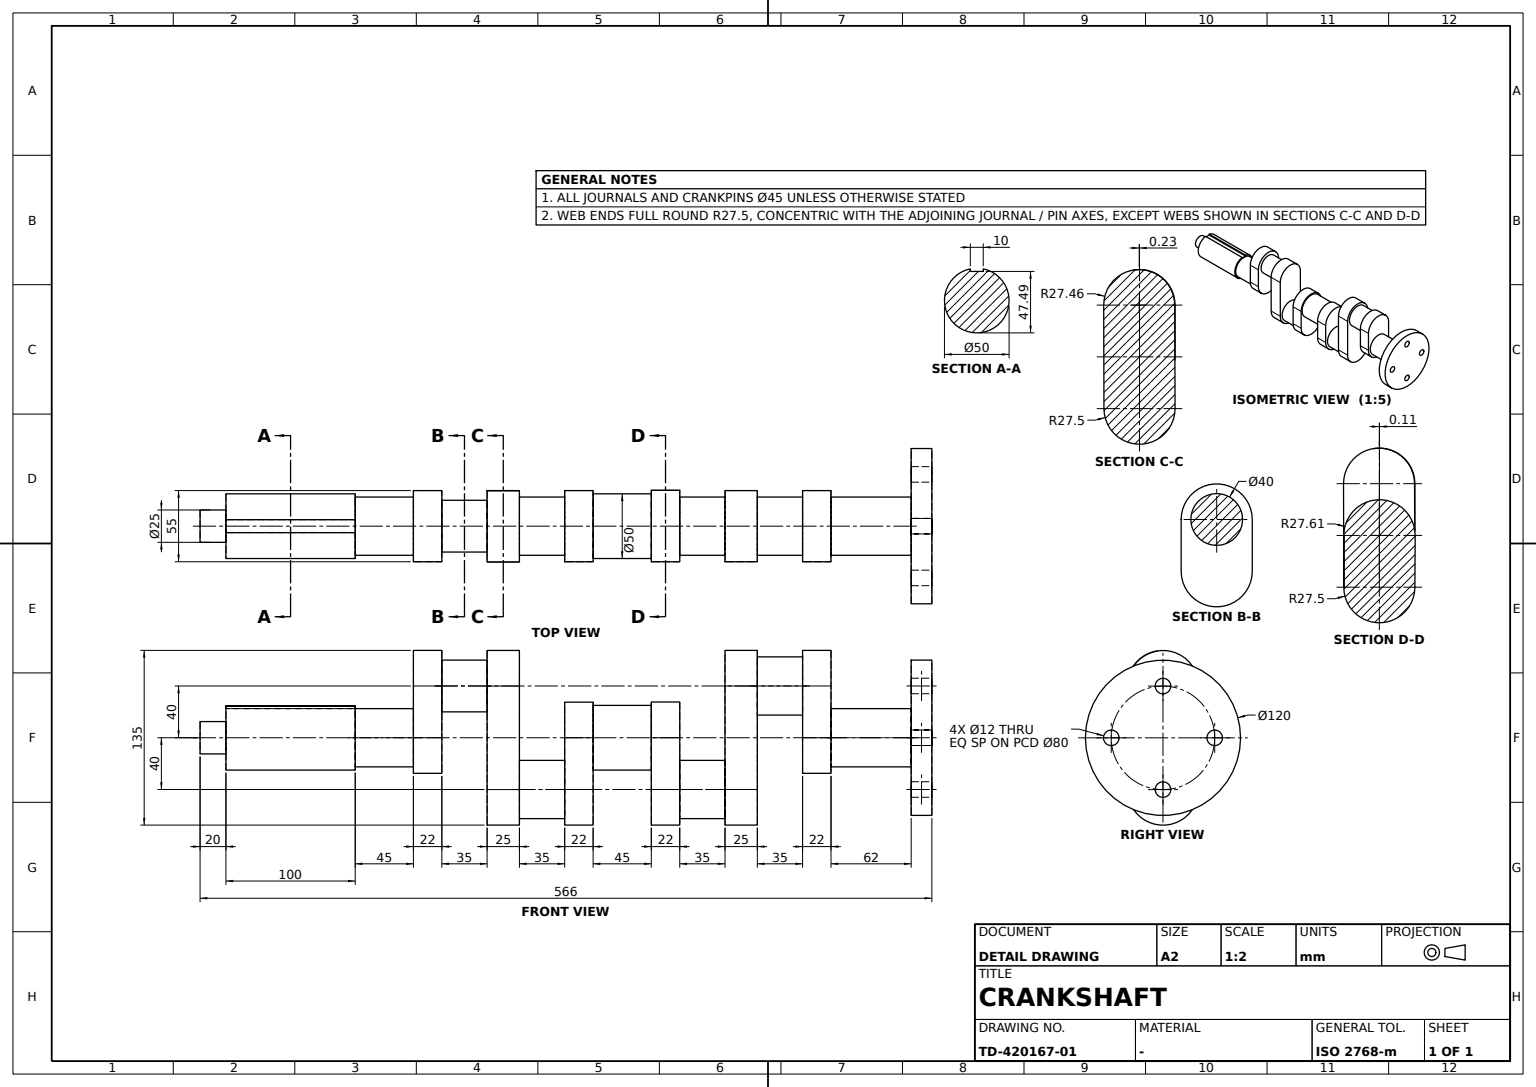
ISO-10303-21;
HEADER;
FILE_DESCRIPTION((''),'2;1');
FILE_NAME('','',(''),(''),'','','');
FILE_SCHEMA(('AUTOMOTIVE_DESIGN'));
ENDSEC;
DATA;
#1=APPLICATION_CONTEXT('');
#2=PRODUCT_CONTEXT('',#1,'mechanical');
#3=PRODUCT('','','',(#2));
#4=PRODUCT_DEFINITION_FORMATION('','',#3);
#5=PRODUCT_DEFINITION_CONTEXT('',#1,'design');
#6=PRODUCT_DEFINITION('','',#4,#5);
#7=PRODUCT_DEFINITION_SHAPE('','',#6);
#8=(LENGTH_UNIT()NAMED_UNIT(*)SI_UNIT(.MILLI.,.METRE.));
#9=(NAMED_UNIT(*)PLANE_ANGLE_UNIT()SI_UNIT($,.RADIAN.));
#10=(NAMED_UNIT(*)SI_UNIT($,.STERADIAN.)SOLID_ANGLE_UNIT());
#11=UNCERTAINTY_MEASURE_WITH_UNIT(LENGTH_MEASURE(0.005),#8,'distance_accuracy_value','');
#12=(GEOMETRIC_REPRESENTATION_CONTEXT(3)GLOBAL_UNCERTAINTY_ASSIGNED_CONTEXT((#11))GLOBAL_UNIT_ASSIGNED_CONTEXT((#8,#9,#10))REPRESENTATION_CONTEXT('',''));
#13=CARTESIAN_POINT('',(-438.,24.494897,-5.));
#14=VERTEX_POINT('',#13);
#15=CARTESIAN_POINT('',(-438.,24.494897,5.));
#16=VERTEX_POINT('',#15);
#17=CARTESIAN_POINT('',(-438.,0.,0.));
#18=DIRECTION('',(-1.,0.,0.));
#19=DIRECTION('',(0.,0.,1.));
#20=AXIS2_PLACEMENT_3D('',#17,#18,#19);
#21=CIRCLE('',#20,25.);
#22=EDGE_CURVE('',#14,#16,#21,.T.);
#23=ORIENTED_EDGE('',*,*,#22,.T.);
#24=CARTESIAN_POINT('',(-538.,24.494897,5.));
#25=VERTEX_POINT('',#24);
#26=VECTOR('',#18,1000.);
#27=LINE('',#24,#26);
#28=EDGE_CURVE('',#25,#16,#27,.F.);
#29=ORIENTED_EDGE('',*,*,#28,.F.);
#30=CARTESIAN_POINT('',(-538.,24.494897,-5.));
#31=VERTEX_POINT('',#30);
#32=CARTESIAN_POINT('',(-538.,0.,0.));
#33=AXIS2_PLACEMENT_3D('',#32,#18,#19);
#34=CIRCLE('',#33,25.);
#35=EDGE_CURVE('',#31,#25,#34,.T.);
#36=ORIENTED_EDGE('',*,*,#35,.F.);
#37=LINE('',#30,#26);
#38=EDGE_CURVE('',#31,#14,#37,.F.);
#39=ORIENTED_EDGE('',*,*,#38,.T.);
#40=EDGE_LOOP('',(#23,#29,#36,#39));
#41=FACE_BOUND('',#40,.T.);
#42=CARTESIAN_POINT('',(-231.5,0.,0.));
#43=DIRECTION('',(0.,-1.,0.));
#44=AXIS2_PLACEMENT_3D('',#42,#18,#43);
#45=CYLINDRICAL_SURFACE('',#44,25.);
#46=ADVANCED_FACE('',(#41),#45,.T.);
#47=CARTESIAN_POINT('',(-254.,0.,27.5));
#48=VERTEX_POINT('',#47);
#49=CARTESIAN_POINT('',(-276.,0.,27.5));
#50=VERTEX_POINT('',#49);
#51=CARTESIAN_POINT('',(-81.,0.,27.5));
#52=LINE('',#51,#26);
#53=EDGE_CURVE('',#48,#50,#52,.T.);
#54=ORIENTED_EDGE('',*,*,#53,.T.);
#55=CARTESIAN_POINT('',(-276.,-40.,27.5));
#56=VERTEX_POINT('',#55);
#57=VECTOR('',#43,1000.);
#58=LINE('',#49,#57);
#59=EDGE_CURVE('',#50,#56,#58,.T.);
#60=ORIENTED_EDGE('',*,*,#59,.T.);
#61=CARTESIAN_POINT('',(-254.,-40.,27.5));
#62=VERTEX_POINT('',#61);
#63=CARTESIAN_POINT('',(-139.5,-40.,27.5));
#64=LINE('',#63,#26);
#65=EDGE_CURVE('',#62,#56,#64,.T.);
#66=ORIENTED_EDGE('',*,*,#65,.F.);
#67=LINE('',#47,#57);
#68=EDGE_CURVE('',#48,#62,#67,.T.);
#69=ORIENTED_EDGE('',*,*,#68,.F.);
#70=EDGE_LOOP('',(#54,#60,#66,#69));
#71=FACE_BOUND('',#70,.T.);
#72=CARTESIAN_POINT('',(-70.,0.,27.5));
#73=DIRECTION('',(0.,1.,0.));
#74=AXIS2_PLACEMENT_3D('',#72,#19,#73);
#75=PLANE('',#74);
#76=ADVANCED_FACE('',(#71),#75,.T.);
#77=CARTESIAN_POINT('',(-311.,39.93292,27.694372));
#78=VERTEX_POINT('',#77);
#79=CARTESIAN_POINT('',(-311.,40.09153,-27.232277));
#80=VERTEX_POINT('',#79);
#81=CARTESIAN_POINT('',(-311.,39.999675,0.231011));
#82=AXIS2_PLACEMENT_3D('',#81,#18,#19);
#83=CIRCLE('',#82,27.463442);
#84=EDGE_CURVE('',#78,#80,#83,.T.);
#85=ORIENTED_EDGE('',*,*,#84,.F.);
#86=CARTESIAN_POINT('',(-311.,-40.066843,27.499919));
#87=VERTEX_POINT('',#86);
#88=CARTESIAN_POINT('',(-311.,-0.06708,27.597145));
#89=DIRECTION('',(0.,0.999997046,0.002430665));
#90=VECTOR('',#89,1000.);
#91=LINE('',#88,#90);
#92=EDGE_CURVE('',#87,#78,#91,.T.);
#93=ORIENTED_EDGE('',*,*,#92,.F.);
#94=CARTESIAN_POINT('',(-311.,-39.908023,-27.499846));
#95=VERTEX_POINT('',#94);
#96=CARTESIAN_POINT('',(-311.,-40.,0.));
#97=AXIS2_PLACEMENT_3D('',#96,#18,#19);
#98=CIRCLE('',#97,27.5);
#99=EDGE_CURVE('',#95,#87,#98,.T.);
#100=ORIENTED_EDGE('',*,*,#99,.F.);
#101=CARTESIAN_POINT('',(-311.,0.09153,-27.366062));
#102=DIRECTION('',(0.,0.999994407,0.003344618));
#103=VECTOR('',#102,1000.);
#104=LINE('',#101,#103);
#105=EDGE_CURVE('',#95,#80,#104,.T.);
#106=ORIENTED_EDGE('',*,*,#105,.T.);
#107=EDGE_LOOP('',(#85,#93,#100,#106));
#108=FACE_BOUND('',#107,.T.);
#109=CARTESIAN_POINT('',(-311.,-40.,22.5));
#110=VERTEX_POINT('',#109);
#111=CIRCLE('',#97,22.5);
#112=EDGE_CURVE('',#110,#110,#111,.T.);
#113=ORIENTED_EDGE('',*,*,#112,.T.);
#114=EDGE_LOOP('',(#113));
#115=FACE_BOUND('',#114,.T.);
#116=CARTESIAN_POINT('',(-311.,0.,0.));
#117=AXIS2_PLACEMENT_3D('',#116,#18,#43);
#118=PLANE('',#117);
#119=ADVANCED_FACE('',(#108,#115),#118,.F.);
#120=CARTESIAN_POINT('',(-70.,-0.005103,22.5));
#121=VERTEX_POINT('',#120);
#122=CARTESIAN_POINT('',(-70.,-0.005103,0.));
#123=AXIS2_PLACEMENT_3D('',#122,#18,#19);
#124=CIRCLE('',#123,22.5);
#125=EDGE_CURVE('',#121,#121,#124,.T.);
#126=ORIENTED_EDGE('',*,*,#125,.T.);
#127=EDGE_LOOP('',(#126));
#128=FACE_BOUND('',#127,.T.);
#129=CARTESIAN_POINT('',(-70.,0.,-27.5));
#130=VERTEX_POINT('',#129);
#131=VERTEX_POINT('',#72);
#132=CARTESIAN_POINT('',(-70.,0.,0.));
#133=AXIS2_PLACEMENT_3D('',#132,#18,#19);
#134=CIRCLE('',#133,27.5);
#135=EDGE_CURVE('',#130,#131,#134,.T.);
#136=ORIENTED_EDGE('',*,*,#135,.F.);
#137=CARTESIAN_POINT('',(-70.,40.,-27.5));
#138=VERTEX_POINT('',#137);
#139=VECTOR('',#73,1000.);
#140=LINE('',#129,#139);
#141=EDGE_CURVE('',#130,#138,#140,.T.);
#142=ORIENTED_EDGE('',*,*,#141,.T.);
#143=CARTESIAN_POINT('',(-70.,40.,27.5));
#144=VERTEX_POINT('',#143);
#145=CARTESIAN_POINT('',(-70.,40.,0.));
#146=AXIS2_PLACEMENT_3D('',#145,#18,#19);
#147=CIRCLE('',#146,27.5);
#148=EDGE_CURVE('',#144,#138,#147,.T.);
#149=ORIENTED_EDGE('',*,*,#148,.F.);
#150=LINE('',#72,#139);
#151=EDGE_CURVE('',#131,#144,#150,.T.);
#152=ORIENTED_EDGE('',*,*,#151,.F.);
#153=EDGE_LOOP('',(#136,#142,#149,#152));
#154=FACE_BOUND('',#153,.T.);
#155=AXIS2_PLACEMENT_3D('',#132,#18,#43);
#156=PLANE('',#155);
#157=ADVANCED_FACE('',(#128,#154),#156,.F.);
#158=CARTESIAN_POINT('',(-92.,40.,27.5));
#159=VERTEX_POINT('',#158);
#160=CARTESIAN_POINT('',(-92.,40.,-27.5));
#161=VERTEX_POINT('',#160);
#162=CARTESIAN_POINT('',(-92.,40.,0.));
#163=AXIS2_PLACEMENT_3D('',#162,#18,#19);
#164=CIRCLE('',#163,27.5);
#165=EDGE_CURVE('',#159,#161,#164,.T.);
#166=ORIENTED_EDGE('',*,*,#165,.F.);
#167=CARTESIAN_POINT('',(-81.,40.,27.5));
#168=LINE('',#167,#26);
#169=EDGE_CURVE('',#144,#159,#168,.T.);
#170=ORIENTED_EDGE('',*,*,#169,.F.);
#171=ORIENTED_EDGE('',*,*,#148,.T.);
#172=CARTESIAN_POINT('',(-81.,40.,-27.5));
#173=LINE('',#172,#26);
#174=EDGE_CURVE('',#138,#161,#173,.T.);
#175=ORIENTED_EDGE('',*,*,#174,.T.);
#176=EDGE_LOOP('',(#166,#170,#171,#175));
#177=FACE_BOUND('',#176,.T.);
#178=CARTESIAN_POINT('',(-81.,40.,0.));
#179=AXIS2_PLACEMENT_3D('',#178,#18,#43);
#180=CYLINDRICAL_SURFACE('',#179,27.5);
#181=ADVANCED_FACE('',(#177),#180,.T.);
#182=CARTESIAN_POINT('',(-438.,22.494897,5.));
#183=VERTEX_POINT('',#182);
#184=CARTESIAN_POINT('',(-438.,22.494897,0.479171));
#185=VERTEX_POINT('',#184);
#186=DIRECTION('',(0.,0.,-1.));
#187=VECTOR('',#186,1000.);
#188=LINE('',#182,#187);
#189=EDGE_CURVE('',#183,#185,#188,.T.);
#190=ORIENTED_EDGE('',*,*,#189,.T.);
#191=CARTESIAN_POINT('',(-438.,22.497449,0.));
#192=VERTEX_POINT('',#191);
#193=CARTESIAN_POINT('',(-438.,22.494897,0.479155));
#194=CARTESIAN_POINT('',(-438.,22.494897,0.319437));
#195=CARTESIAN_POINT('',(-438.,22.494897,0.159718));
#196=CARTESIAN_POINT('',(-438.,22.494897,0.));
#197=B_SPLINE_CURVE_WITH_KNOTS('',3,(#193,#194,#195,#196),.UNSPECIFIED.,.F.,.F.,(4,4),(4.520844794,5.),.UNSPECIFIED.);
#198=EDGE_CURVE('',#185,#192,#197,.T.);
#199=ORIENTED_EDGE('',*,*,#198,.T.);
#200=CARTESIAN_POINT('',(-438.,22.494897,-0.479171));
#201=VERTEX_POINT('',#200);
#202=CARTESIAN_POINT('',(-438.,22.494897,-0.159718));
#203=CARTESIAN_POINT('',(-438.,22.494897,-0.319437));
#204=CARTESIAN_POINT('',(-438.,22.494897,-0.479155));
#205=B_SPLINE_CURVE_WITH_KNOTS('',3,(#196,#202,#203,#204),.UNSPECIFIED.,.F.,.F.,(4,4),(5.,5.479155206),.UNSPECIFIED.);
#206=EDGE_CURVE('',#192,#201,#205,.T.);
#207=ORIENTED_EDGE('',*,*,#206,.T.);
#208=CARTESIAN_POINT('',(-438.,22.494897,-5.));
#209=VERTEX_POINT('',#208);
#210=EDGE_CURVE('',#201,#209,#188,.T.);
#211=ORIENTED_EDGE('',*,*,#210,.T.);
#212=CARTESIAN_POINT('',(-538.,22.494897,-5.));
#213=VERTEX_POINT('',#212);
#214=DIRECTION('',(1.,0.,0.));
#215=VECTOR('',#214,1000.);
#216=LINE('',#212,#215);
#217=EDGE_CURVE('',#213,#209,#216,.T.);
#218=ORIENTED_EDGE('',*,*,#217,.F.);
#219=CARTESIAN_POINT('',(-538.,22.494897,5.));
#220=VERTEX_POINT('',#219);
#221=LINE('',#219,#187);
#222=EDGE_CURVE('',#220,#213,#221,.T.);
#223=ORIENTED_EDGE('',*,*,#222,.F.);
#224=LINE('',#219,#215);
#225=EDGE_CURVE('',#220,#183,#224,.T.);
#226=ORIENTED_EDGE('',*,*,#225,.T.);
#227=EDGE_LOOP('',(#190,#199,#207,#211,#218,#223,#226));
#228=FACE_BOUND('',#227,.T.);
#229=AXIS2_PLACEMENT_3D('',#219,#43,#186);
#230=PLANE('',#229);
#231=ADVANCED_FACE('',(#228),#230,.F.);
#232=CARTESIAN_POINT('',(8.,0.,-46.));
#233=VERTEX_POINT('',#232);
#234=CARTESIAN_POINT('',(8.,0.,-40.));
#235=AXIS2_PLACEMENT_3D('',#234,#214,#186);
#236=CIRCLE('',#235,6.);
#237=EDGE_CURVE('',#233,#233,#236,.T.);
#238=ORIENTED_EDGE('',*,*,#237,.F.);
#239=EDGE_LOOP('',(#238));
#240=FACE_BOUND('',#239,.T.);
#241=CARTESIAN_POINT('',(8.,-40.,-6.));
#242=VERTEX_POINT('',#241);
#243=CARTESIAN_POINT('',(8.,-40.,0.));
#244=AXIS2_PLACEMENT_3D('',#243,#214,#186);
#245=CIRCLE('',#244,6.);
#246=EDGE_CURVE('',#242,#242,#245,.T.);
#247=ORIENTED_EDGE('',*,*,#246,.F.);
#248=EDGE_LOOP('',(#247));
#249=FACE_BOUND('',#248,.T.);
#250=CARTESIAN_POINT('',(8.,0.,34.));
#251=VERTEX_POINT('',#250);
#252=CARTESIAN_POINT('',(8.,0.,40.));
#253=AXIS2_PLACEMENT_3D('',#252,#214,#186);
#254=CIRCLE('',#253,6.);
#255=EDGE_CURVE('',#251,#251,#254,.T.);
#256=ORIENTED_EDGE('',*,*,#255,.F.);
#257=EDGE_LOOP('',(#256));
#258=FACE_BOUND('',#257,.T.);
#259=CARTESIAN_POINT('',(8.,0.,-60.));
#260=VERTEX_POINT('',#259);
#261=CARTESIAN_POINT('',(8.,0.,0.));
#262=AXIS2_PLACEMENT_3D('',#261,#214,#186);
#263=CIRCLE('',#262,60.);
#264=EDGE_CURVE('',#260,#260,#263,.T.);
#265=ORIENTED_EDGE('',*,*,#264,.T.);
#266=EDGE_LOOP('',(#265));
#267=FACE_BOUND('',#266,.T.);
#268=CARTESIAN_POINT('',(8.,40.,-6.));
#269=VERTEX_POINT('',#268);
#270=CARTESIAN_POINT('',(8.,40.,0.));
#271=AXIS2_PLACEMENT_3D('',#270,#214,#186);
#272=CIRCLE('',#271,6.);
#273=EDGE_CURVE('',#269,#269,#272,.T.);
#274=ORIENTED_EDGE('',*,*,#273,.F.);
#275=EDGE_LOOP('',(#274));
#276=FACE_BOUND('',#275,.T.);
#277=AXIS2_PLACEMENT_3D('',#261,#214,#73);
#278=PLANE('',#277);
#279=ADVANCED_FACE('',(#240,#249,#258,#267,#276),#278,.T.);
#280=CARTESIAN_POINT('',(-371.,0.,-27.5));
#281=VERTEX_POINT('',#280);
#282=CARTESIAN_POINT('',(-371.,0.,27.5));
#283=VERTEX_POINT('',#282);
#284=CARTESIAN_POINT('',(-371.,0.,0.));
#285=AXIS2_PLACEMENT_3D('',#284,#18,#19);
#286=CIRCLE('',#285,27.5);
#287=EDGE_CURVE('',#281,#283,#286,.T.);
#288=ORIENTED_EDGE('',*,*,#287,.T.);
#289=CARTESIAN_POINT('',(-393.,0.,27.5));
#290=VERTEX_POINT('',#289);
#291=EDGE_CURVE('',#283,#290,#52,.T.);
#292=ORIENTED_EDGE('',*,*,#291,.T.);
#293=CARTESIAN_POINT('',(-393.,0.,-27.5));
#294=VERTEX_POINT('',#293);
#295=CARTESIAN_POINT('',(-393.,0.,0.));
#296=AXIS2_PLACEMENT_3D('',#295,#18,#19);
#297=CIRCLE('',#296,27.5);
#298=EDGE_CURVE('',#294,#290,#297,.T.);
#299=ORIENTED_EDGE('',*,*,#298,.F.);
#300=CARTESIAN_POINT('',(-81.,0.,-27.5));
#301=LINE('',#300,#26);
#302=EDGE_CURVE('',#281,#294,#301,.T.);
#303=ORIENTED_EDGE('',*,*,#302,.F.);
#304=EDGE_LOOP('',(#288,#292,#299,#303));
#305=FACE_BOUND('',#304,.T.);
#306=CARTESIAN_POINT('',(-81.,0.,0.));
#307=AXIS2_PLACEMENT_3D('',#306,#18,#43);
#308=CYLINDRICAL_SURFACE('',#307,27.5);
#309=ADVANCED_FACE('',(#305),#308,.T.);
#310=CARTESIAN_POINT('',(-336.,40.,20.));
#311=VERTEX_POINT('',#310);
#312=CARTESIAN_POINT('',(-336.,40.,0.));
#313=AXIS2_PLACEMENT_3D('',#312,#18,#19);
#314=CIRCLE('',#313,20.);
#315=EDGE_CURVE('',#311,#311,#314,.T.);
#316=ORIENTED_EDGE('',*,*,#315,.F.);
#317=EDGE_LOOP('',(#316));
#318=FACE_BOUND('',#317,.T.);
#319=CARTESIAN_POINT('',(-336.,-39.908023,-27.499846));
#320=VERTEX_POINT('',#319);
#321=CARTESIAN_POINT('',(-336.,-40.066843,27.499919));
#322=VERTEX_POINT('',#321);
#323=CARTESIAN_POINT('',(-336.,-40.,0.));
#324=AXIS2_PLACEMENT_3D('',#323,#18,#19);
#325=CIRCLE('',#324,27.5);
#326=EDGE_CURVE('',#320,#322,#325,.T.);
#327=ORIENTED_EDGE('',*,*,#326,.T.);
#328=CARTESIAN_POINT('',(-336.,39.93292,27.694372));
#329=VERTEX_POINT('',#328);
#330=CARTESIAN_POINT('',(-336.,-0.06708,27.597145));
#331=LINE('',#330,#90);
#332=EDGE_CURVE('',#322,#329,#331,.T.);
#333=ORIENTED_EDGE('',*,*,#332,.T.);
#334=CARTESIAN_POINT('',(-336.,40.09153,-27.232277));
#335=VERTEX_POINT('',#334);
#336=CARTESIAN_POINT('',(-336.,39.999675,0.231011));
#337=AXIS2_PLACEMENT_3D('',#336,#18,#19);
#338=CIRCLE('',#337,27.463442);
#339=EDGE_CURVE('',#329,#335,#338,.T.);
#340=ORIENTED_EDGE('',*,*,#339,.T.);
#341=CARTESIAN_POINT('',(-336.,0.09153,-27.366062));
#342=LINE('',#341,#103);
#343=EDGE_CURVE('',#320,#335,#342,.T.);
#344=ORIENTED_EDGE('',*,*,#343,.F.);
#345=EDGE_LOOP('',(#327,#333,#340,#344));
#346=FACE_BOUND('',#345,.T.);
#347=CARTESIAN_POINT('',(-336.,0.,0.));
#348=AXIS2_PLACEMENT_3D('',#347,#18,#43);
#349=PLANE('',#348);
#350=ADVANCED_FACE('',(#318,#346),#349,.T.);
#351=CARTESIAN_POINT('',(-538.,0.,12.5));
#352=VERTEX_POINT('',#351);
#353=CIRCLE('',#33,12.5);
#354=EDGE_CURVE('',#352,#352,#353,.T.);
#355=ORIENTED_EDGE('',*,*,#354,.T.);
#356=EDGE_LOOP('',(#355));
#357=FACE_BOUND('',#356,.T.);
#358=CARTESIAN_POINT('',(-558.,0.,12.5));
#359=VERTEX_POINT('',#358);
#360=CARTESIAN_POINT('',(-558.,0.,0.));
#361=AXIS2_PLACEMENT_3D('',#360,#18,#19);
#362=CIRCLE('',#361,12.5);
#363=EDGE_CURVE('',#359,#359,#362,.T.);
#364=ORIENTED_EDGE('',*,*,#363,.F.);
#365=EDGE_LOOP('',(#364));
#366=FACE_BOUND('',#365,.T.);
#367=CARTESIAN_POINT('',(-548.,0.,0.));
#368=AXIS2_PLACEMENT_3D('',#367,#18,#43);
#369=CYLINDRICAL_SURFACE('',#368,12.5);
#370=ADVANCED_FACE('',(#357,#366),#369,.T.);
#371=ORIENTED_EDGE('',*,*,#38,.F.);
#372=LINE('',#212,#139);
#373=EDGE_CURVE('',#213,#31,#372,.T.);
#374=ORIENTED_EDGE('',*,*,#373,.F.);
#375=ORIENTED_EDGE('',*,*,#217,.T.);
#376=LINE('',#208,#139);
#377=EDGE_CURVE('',#209,#14,#376,.T.);
#378=ORIENTED_EDGE('',*,*,#377,.T.);
#379=EDGE_LOOP('',(#371,#374,#375,#378));
#380=FACE_BOUND('',#379,.T.);
#381=AXIS2_PLACEMENT_3D('',#212,#186,#73);
#382=PLANE('',#381);
#383=ADVANCED_FACE('',(#380),#382,.F.);
#384=CARTESIAN_POINT('',(-8.,40.,-6.));
#385=VERTEX_POINT('',#384);
#386=CARTESIAN_POINT('',(-8.,40.,0.));
#387=AXIS2_PLACEMENT_3D('',#386,#214,#186);
#388=CIRCLE('',#387,6.);
#389=EDGE_CURVE('',#385,#385,#388,.T.);
#390=ORIENTED_EDGE('',*,*,#389,.F.);
#391=EDGE_LOOP('',(#390));
#392=FACE_BOUND('',#391,.T.);
#393=ORIENTED_EDGE('',*,*,#273,.T.);
#394=EDGE_LOOP('',(#393));
#395=FACE_BOUND('',#394,.T.);
#396=CARTESIAN_POINT('',(0.,40.,0.));
#397=AXIS2_PLACEMENT_3D('',#396,#214,#73);
#398=CYLINDRICAL_SURFACE('',#397,6.);
#399=ADVANCED_FACE('',(#392,#395),#398,.F.);
#400=CARTESIAN_POINT('',(-187.,-40.,22.5));
#401=VERTEX_POINT('',#400);
#402=CARTESIAN_POINT('',(-187.,-40.,0.));
#403=AXIS2_PLACEMENT_3D('',#402,#18,#19);
#404=CIRCLE('',#403,22.5);
#405=EDGE_CURVE('',#401,#401,#404,.T.);
#406=ORIENTED_EDGE('',*,*,#405,.F.);
#407=EDGE_LOOP('',(#406));
#408=FACE_BOUND('',#407,.T.);
#409=CARTESIAN_POINT('',(-152.,-40.,22.5));
#410=VERTEX_POINT('',#409);
#411=CARTESIAN_POINT('',(-152.,-40.,0.));
#412=AXIS2_PLACEMENT_3D('',#411,#18,#19);
#413=CIRCLE('',#412,22.5);
#414=EDGE_CURVE('',#410,#410,#413,.T.);
#415=ORIENTED_EDGE('',*,*,#414,.T.);
#416=EDGE_LOOP('',(#415));
#417=FACE_BOUND('',#416,.T.);
#418=CARTESIAN_POINT('',(-169.5,-40.,0.));
#419=AXIS2_PLACEMENT_3D('',#418,#18,#43);
#420=CYLINDRICAL_SURFACE('',#419,22.5);
#421=ADVANCED_FACE('',(#408,#417),#420,.T.);
#422=CARTESIAN_POINT('',(-371.,40.,-27.5));
#423=VERTEX_POINT('',#422);
#424=CARTESIAN_POINT('',(-393.,40.,-27.5));
#425=VERTEX_POINT('',#424);
#426=EDGE_CURVE('',#423,#425,#173,.T.);
#427=ORIENTED_EDGE('',*,*,#426,.T.);
#428=CARTESIAN_POINT('',(-393.,40.,27.5));
#429=VERTEX_POINT('',#428);
#430=CARTESIAN_POINT('',(-393.,40.,0.));
#431=AXIS2_PLACEMENT_3D('',#430,#18,#19);
#432=CIRCLE('',#431,27.5);
#433=EDGE_CURVE('',#429,#425,#432,.T.);
#434=ORIENTED_EDGE('',*,*,#433,.F.);
#435=CARTESIAN_POINT('',(-371.,40.,27.5));
#436=VERTEX_POINT('',#435);
#437=EDGE_CURVE('',#436,#429,#168,.T.);
#438=ORIENTED_EDGE('',*,*,#437,.F.);
#439=CARTESIAN_POINT('',(-371.,40.,0.));
#440=AXIS2_PLACEMENT_3D('',#439,#18,#19);
#441=CIRCLE('',#440,27.5);
#442=EDGE_CURVE('',#436,#423,#441,.T.);
#443=ORIENTED_EDGE('',*,*,#442,.T.);
#444=EDGE_LOOP('',(#427,#434,#438,#443));
#445=FACE_BOUND('',#444,.T.);
#446=ADVANCED_FACE('',(#445),#180,.T.);
#447=CARTESIAN_POINT('',(-393.,-0.005103,22.5));
#448=VERTEX_POINT('',#447);
#449=CARTESIAN_POINT('',(-393.,-0.005103,0.));
#450=AXIS2_PLACEMENT_3D('',#449,#18,#19);
#451=CIRCLE('',#450,22.5);
#452=EDGE_CURVE('',#448,#448,#451,.T.);
#453=ORIENTED_EDGE('',*,*,#452,.T.);
#454=EDGE_LOOP('',(#453));
#455=FACE_BOUND('',#454,.T.);
#456=CARTESIAN_POINT('',(-438.,-0.005103,0.));
#457=AXIS2_PLACEMENT_3D('',#456,#18,#19);
#458=CIRCLE('',#457,22.5);
#459=EDGE_CURVE('',#201,#185,#458,.T.);
#460=ORIENTED_EDGE('',*,*,#459,.F.);
#461=ORIENTED_EDGE('',*,*,#206,.F.);
#462=ORIENTED_EDGE('',*,*,#198,.F.);
#463=EDGE_LOOP('',(#460,#461,#462));
#464=FACE_BOUND('',#463,.T.);
#465=CARTESIAN_POINT('',(-39.,-0.005103,0.));
#466=AXIS2_PLACEMENT_3D('',#465,#18,#43);
#467=CYLINDRICAL_SURFACE('',#466,22.5);
#468=ADVANCED_FACE('',(#455,#464),#467,.T.);
#469=CARTESIAN_POINT('',(-209.,0.,25.));
#470=VERTEX_POINT('',#469);
#471=CARTESIAN_POINT('',(-209.,0.,0.));
#472=AXIS2_PLACEMENT_3D('',#471,#18,#19);
#473=CIRCLE('',#472,25.);
#474=EDGE_CURVE('',#470,#470,#473,.T.);
#475=ORIENTED_EDGE('',*,*,#474,.T.);
#476=EDGE_LOOP('',(#475));
#477=FACE_BOUND('',#476,.T.);
#478=CARTESIAN_POINT('',(-254.,0.,25.));
#479=VERTEX_POINT('',#478);
#480=CARTESIAN_POINT('',(-254.,0.,0.));
#481=AXIS2_PLACEMENT_3D('',#480,#18,#19);
#482=CIRCLE('',#481,25.);
#483=EDGE_CURVE('',#479,#479,#482,.T.);
#484=ORIENTED_EDGE('',*,*,#483,.F.);
#485=EDGE_LOOP('',(#484));
#486=FACE_BOUND('',#485,.T.);
#487=ADVANCED_FACE('',(#477,#486),#45,.T.);
#488=CARTESIAN_POINT('',(-371.,40.,20.));
#489=VERTEX_POINT('',#488);
#490=CIRCLE('',#440,20.);
#491=EDGE_CURVE('',#489,#489,#490,.T.);
#492=ORIENTED_EDGE('',*,*,#491,.T.);
#493=EDGE_LOOP('',(#492));
#494=FACE_BOUND('',#493,.T.);
#495=ORIENTED_EDGE('',*,*,#287,.F.);
#496=LINE('',#280,#57);
#497=EDGE_CURVE('',#423,#281,#496,.T.);
#498=ORIENTED_EDGE('',*,*,#497,.F.);
#499=ORIENTED_EDGE('',*,*,#442,.F.);
#500=LINE('',#282,#57);
#501=EDGE_CURVE('',#436,#283,#500,.T.);
#502=ORIENTED_EDGE('',*,*,#501,.T.);
#503=EDGE_LOOP('',(#495,#498,#499,#502));
#504=FACE_BOUND('',#503,.T.);
#505=AXIS2_PLACEMENT_3D('',#284,#18,#43);
#506=PLANE('',#505);
#507=ADVANCED_FACE('',(#494,#504),#506,.F.);
#508=CARTESIAN_POINT('',(-254.,-40.,-27.5));
#509=VERTEX_POINT('',#508);
#510=CARTESIAN_POINT('',(-276.,-40.,-27.5));
#511=VERTEX_POINT('',#510);
#512=CARTESIAN_POINT('',(-139.5,-40.,-27.5));
#513=LINE('',#512,#26);
#514=EDGE_CURVE('',#509,#511,#513,.T.);
#515=ORIENTED_EDGE('',*,*,#514,.F.);
#516=CARTESIAN_POINT('',(-254.,-40.,0.));
#517=AXIS2_PLACEMENT_3D('',#516,#18,#19);
#518=CIRCLE('',#517,27.5);
#519=EDGE_CURVE('',#509,#62,#518,.T.);
#520=ORIENTED_EDGE('',*,*,#519,.T.);
#521=ORIENTED_EDGE('',*,*,#65,.T.);
#522=CARTESIAN_POINT('',(-276.,-40.,0.));
#523=AXIS2_PLACEMENT_3D('',#522,#18,#19);
#524=CIRCLE('',#523,27.5);
#525=EDGE_CURVE('',#511,#56,#524,.T.);
#526=ORIENTED_EDGE('',*,*,#525,.F.);
#527=EDGE_LOOP('',(#515,#520,#521,#526));
#528=FACE_BOUND('',#527,.T.);
#529=CARTESIAN_POINT('',(-139.5,-40.,0.));
#530=AXIS2_PLACEMENT_3D('',#529,#18,#43);
#531=CYLINDRICAL_SURFACE('',#530,27.5);
#532=ADVANCED_FACE('',(#528),#531,.T.);
#533=ORIENTED_EDGE('',*,*,#225,.F.);
#534=LINE('',#24,#57);
#535=EDGE_CURVE('',#25,#220,#534,.T.);
#536=ORIENTED_EDGE('',*,*,#535,.F.);
#537=ORIENTED_EDGE('',*,*,#28,.T.);
#538=LINE('',#15,#57);
#539=EDGE_CURVE('',#16,#183,#538,.T.);
#540=ORIENTED_EDGE('',*,*,#539,.T.);
#541=EDGE_LOOP('',(#533,#536,#537,#540));
#542=FACE_BOUND('',#541,.T.);
#543=AXIS2_PLACEMENT_3D('',#24,#19,#43);
#544=PLANE('',#543);
#545=ADVANCED_FACE('',(#542),#544,.F.);
#546=CARTESIAN_POINT('',(-276.,0.,-27.5));
#547=VERTEX_POINT('',#546);
#548=CARTESIAN_POINT('',(-276.,0.,0.));
#549=AXIS2_PLACEMENT_3D('',#548,#18,#19);
#550=CIRCLE('',#549,27.5);
#551=EDGE_CURVE('',#50,#547,#550,.T.);
#552=ORIENTED_EDGE('',*,*,#551,.F.);
#553=ORIENTED_EDGE('',*,*,#53,.F.);
#554=CARTESIAN_POINT('',(-254.,0.,-27.5));
#555=VERTEX_POINT('',#554);
#556=CIRCLE('',#481,27.5);
#557=EDGE_CURVE('',#48,#555,#556,.T.);
#558=ORIENTED_EDGE('',*,*,#557,.T.);
#559=EDGE_CURVE('',#555,#547,#301,.T.);
#560=ORIENTED_EDGE('',*,*,#559,.T.);
#561=EDGE_LOOP('',(#552,#553,#558,#560));
#562=FACE_BOUND('',#561,.T.);
#563=ADVANCED_FACE('',(#562),#308,.T.);
#564=CARTESIAN_POINT('',(-8.,-0.005103,-22.5));
#565=VERTEX_POINT('',#564);
#566=CARTESIAN_POINT('',(-8.,-0.005103,0.));
#567=AXIS2_PLACEMENT_3D('',#566,#214,#186);
#568=CIRCLE('',#567,22.5);
#569=EDGE_CURVE('',#565,#565,#568,.F.);
#570=ORIENTED_EDGE('',*,*,#569,.F.);
#571=EDGE_LOOP('',(#570));
#572=FACE_BOUND('',#571,.T.);
#573=CARTESIAN_POINT('',(-8.,0.,-60.));
#574=VERTEX_POINT('',#573);
#575=CARTESIAN_POINT('',(-8.,0.,0.));
#576=AXIS2_PLACEMENT_3D('',#575,#214,#186);
#577=CIRCLE('',#576,60.);
#578=EDGE_CURVE('',#574,#574,#577,.T.);
#579=ORIENTED_EDGE('',*,*,#578,.F.);
#580=EDGE_LOOP('',(#579));
#581=FACE_BOUND('',#580,.T.);
#582=CARTESIAN_POINT('',(-8.,0.,-46.));
#583=VERTEX_POINT('',#582);
#584=CARTESIAN_POINT('',(-8.,0.,-40.));
#585=AXIS2_PLACEMENT_3D('',#584,#214,#186);
#586=CIRCLE('',#585,6.);
#587=EDGE_CURVE('',#583,#583,#586,.T.);
#588=ORIENTED_EDGE('',*,*,#587,.T.);
#589=EDGE_LOOP('',(#588));
#590=FACE_BOUND('',#589,.T.);
#591=ORIENTED_EDGE('',*,*,#389,.T.);
#592=EDGE_LOOP('',(#591));
#593=FACE_BOUND('',#592,.T.);
#594=CARTESIAN_POINT('',(-8.,-40.,-6.));
#595=VERTEX_POINT('',#594);
#596=CARTESIAN_POINT('',(-8.,-40.,0.));
#597=AXIS2_PLACEMENT_3D('',#596,#214,#186);
#598=CIRCLE('',#597,6.);
#599=EDGE_CURVE('',#595,#595,#598,.T.);
#600=ORIENTED_EDGE('',*,*,#599,.T.);
#601=EDGE_LOOP('',(#600));
#602=FACE_BOUND('',#601,.T.);
#603=CARTESIAN_POINT('',(-8.,0.,34.));
#604=VERTEX_POINT('',#603);
#605=CARTESIAN_POINT('',(-8.,0.,40.));
#606=AXIS2_PLACEMENT_3D('',#605,#214,#186);
#607=CIRCLE('',#606,6.);
#608=EDGE_CURVE('',#604,#604,#607,.T.);
#609=ORIENTED_EDGE('',*,*,#608,.T.);
#610=EDGE_LOOP('',(#609));
#611=FACE_BOUND('',#610,.T.);
#612=AXIS2_PLACEMENT_3D('',#575,#214,#73);
#613=PLANE('',#612);
#614=ADVANCED_FACE('',(#572,#581,#590,#593,#602,#611),#613,.F.);
#615=CARTESIAN_POINT('',(-139.5,-40.066843,27.499919));
#616=LINE('',#615,#26);
#617=EDGE_CURVE('',#87,#322,#616,.T.);
#618=ORIENTED_EDGE('',*,*,#617,.T.);
#619=ORIENTED_EDGE('',*,*,#326,.F.);
#620=CARTESIAN_POINT('',(-139.5,-39.908023,-27.499846));
#621=LINE('',#620,#26);
#622=EDGE_CURVE('',#95,#320,#621,.T.);
#623=ORIENTED_EDGE('',*,*,#622,.F.);
#624=ORIENTED_EDGE('',*,*,#99,.T.);
#625=EDGE_LOOP('',(#618,#619,#623,#624));
#626=FACE_BOUND('',#625,.T.);
#627=ADVANCED_FACE('',(#626),#531,.T.);
#628=ORIENTED_EDGE('',*,*,#264,.F.);
#629=EDGE_LOOP('',(#628));
#630=FACE_BOUND('',#629,.T.);
#631=ORIENTED_EDGE('',*,*,#578,.T.);
#632=EDGE_LOOP('',(#631));
#633=FACE_BOUND('',#632,.T.);
#634=CARTESIAN_POINT('',(0.,0.,0.));
#635=AXIS2_PLACEMENT_3D('',#634,#214,#73);
#636=CYLINDRICAL_SURFACE('',#635,60.);
#637=ADVANCED_FACE('',(#630,#633),#636,.T.);
#638=ORIENTED_EDGE('',*,*,#599,.F.);
#639=EDGE_LOOP('',(#638));
#640=FACE_BOUND('',#639,.T.);
#641=ORIENTED_EDGE('',*,*,#246,.T.);
#642=EDGE_LOOP('',(#641));
#643=FACE_BOUND('',#642,.T.);
#644=CARTESIAN_POINT('',(0.,-40.,0.));
#645=AXIS2_PLACEMENT_3D('',#644,#214,#73);
#646=CYLINDRICAL_SURFACE('',#645,6.);
#647=ADVANCED_FACE('',(#640,#643),#646,.F.);
#648=ORIENTED_EDGE('',*,*,#426,.F.);
#649=ORIENTED_EDGE('',*,*,#497,.T.);
#650=ORIENTED_EDGE('',*,*,#302,.T.);
#651=LINE('',#293,#57);
#652=EDGE_CURVE('',#425,#294,#651,.T.);
#653=ORIENTED_EDGE('',*,*,#652,.F.);
#654=EDGE_LOOP('',(#648,#649,#650,#653));
#655=FACE_BOUND('',#654,.T.);
#656=AXIS2_PLACEMENT_3D('',#129,#19,#73);
#657=PLANE('',#656);
#658=ADVANCED_FACE('',(#655),#657,.F.);
#659=ORIENTED_EDGE('',*,*,#414,.F.);
#660=EDGE_LOOP('',(#659));
#661=FACE_BOUND('',#660,.T.);
#662=CARTESIAN_POINT('',(-152.,40.,-27.5));
#663=VERTEX_POINT('',#662);
#664=CARTESIAN_POINT('',(-152.,-40.,-27.5));
#665=VERTEX_POINT('',#664);
#666=CARTESIAN_POINT('',(-152.,0.,-27.5));
#667=LINE('',#666,#57);
#668=EDGE_CURVE('',#663,#665,#667,.T.);
#669=ORIENTED_EDGE('',*,*,#668,.T.);
#670=CARTESIAN_POINT('',(-152.,-40.,27.5));
#671=VERTEX_POINT('',#670);
#672=CIRCLE('',#412,27.5);
#673=EDGE_CURVE('',#665,#671,#672,.T.);
#674=ORIENTED_EDGE('',*,*,#673,.T.);
#675=CARTESIAN_POINT('',(-152.,40.,27.5));
#676=VERTEX_POINT('',#675);
#677=CARTESIAN_POINT('',(-152.,0.,27.5));
#678=LINE('',#677,#57);
#679=EDGE_CURVE('',#676,#671,#678,.T.);
#680=ORIENTED_EDGE('',*,*,#679,.F.);
#681=CARTESIAN_POINT('',(-152.,40.,0.));
#682=AXIS2_PLACEMENT_3D('',#681,#18,#19);
#683=CIRCLE('',#682,27.5);
#684=EDGE_CURVE('',#676,#663,#683,.T.);
#685=ORIENTED_EDGE('',*,*,#684,.T.);
#686=EDGE_LOOP('',(#669,#674,#680,#685));
#687=FACE_BOUND('',#686,.T.);
#688=CARTESIAN_POINT('',(-152.,0.,0.));
#689=AXIS2_PLACEMENT_3D('',#688,#18,#43);
#690=PLANE('',#689);
#691=ADVANCED_FACE('',(#661,#687),#690,.T.);
#692=ORIENTED_EDGE('',*,*,#525,.T.);
#693=ORIENTED_EDGE('',*,*,#59,.F.);
#694=ORIENTED_EDGE('',*,*,#551,.T.);
#695=LINE('',#546,#57);
#696=EDGE_CURVE('',#547,#511,#695,.T.);
#697=ORIENTED_EDGE('',*,*,#696,.T.);
#698=EDGE_LOOP('',(#692,#693,#694,#697));
#699=FACE_BOUND('',#698,.T.);
#700=CARTESIAN_POINT('',(-276.,-40.,22.5));
#701=VERTEX_POINT('',#700);
#702=CIRCLE('',#523,22.5);
#703=EDGE_CURVE('',#701,#701,#702,.T.);
#704=ORIENTED_EDGE('',*,*,#703,.F.);
#705=EDGE_LOOP('',(#704));
#706=FACE_BOUND('',#705,.T.);
#707=AXIS2_PLACEMENT_3D('',#548,#18,#43);
#708=PLANE('',#707);
#709=ADVANCED_FACE('',(#699,#706),#708,.T.);
#710=ORIENTED_EDGE('',*,*,#679,.T.);
#711=CARTESIAN_POINT('',(-127.,-40.,27.5));
#712=VERTEX_POINT('',#711);
#713=EDGE_CURVE('',#712,#671,#64,.T.);
#714=ORIENTED_EDGE('',*,*,#713,.F.);
#715=CARTESIAN_POINT('',(-127.,40.,27.5));
#716=VERTEX_POINT('',#715);
#717=CARTESIAN_POINT('',(-127.,0.,27.5));
#718=LINE('',#717,#57);
#719=EDGE_CURVE('',#716,#712,#718,.T.);
#720=ORIENTED_EDGE('',*,*,#719,.F.);
#721=EDGE_CURVE('',#716,#676,#168,.T.);
#722=ORIENTED_EDGE('',*,*,#721,.T.);
#723=EDGE_LOOP('',(#710,#714,#720,#722));
#724=FACE_BOUND('',#723,.T.);
#725=ADVANCED_FACE('',(#724),#75,.T.);
#726=LINE('',#554,#57);
#727=EDGE_CURVE('',#555,#509,#726,.T.);
#728=ORIENTED_EDGE('',*,*,#727,.T.);
#729=ORIENTED_EDGE('',*,*,#514,.T.);
#730=ORIENTED_EDGE('',*,*,#696,.F.);
#731=ORIENTED_EDGE('',*,*,#559,.F.);
#732=EDGE_LOOP('',(#728,#729,#730,#731));
#733=FACE_BOUND('',#732,.T.);
#734=ADVANCED_FACE('',(#733),#657,.F.);
#735=ORIENTED_EDGE('',*,*,#491,.F.);
#736=EDGE_LOOP('',(#735));
#737=FACE_BOUND('',#736,.T.);
#738=ORIENTED_EDGE('',*,*,#315,.T.);
#739=EDGE_LOOP('',(#738));
#740=FACE_BOUND('',#739,.T.);
#741=CARTESIAN_POINT('',(-353.5,40.,0.));
#742=AXIS2_PLACEMENT_3D('',#741,#18,#43);
#743=CYLINDRICAL_SURFACE('',#742,20.);
#744=ADVANCED_FACE('',(#737,#740),#743,.T.);
#745=CARTESIAN_POINT('',(-187.,-40.,27.5));
#746=VERTEX_POINT('',#745);
#747=CARTESIAN_POINT('',(-209.,-40.,27.5));
#748=VERTEX_POINT('',#747);
#749=EDGE_CURVE('',#746,#748,#64,.T.);
#750=ORIENTED_EDGE('',*,*,#749,.F.);
#751=CARTESIAN_POINT('',(-187.,0.,27.5));
#752=VERTEX_POINT('',#751);
#753=LINE('',#751,#57);
#754=EDGE_CURVE('',#752,#746,#753,.T.);
#755=ORIENTED_EDGE('',*,*,#754,.F.);
#756=CARTESIAN_POINT('',(-209.,0.,27.5));
#757=VERTEX_POINT('',#756);
#758=CARTESIAN_POINT('',(-198.,0.,27.5));
#759=LINE('',#758,#26);
#760=EDGE_CURVE('',#752,#757,#759,.T.);
#761=ORIENTED_EDGE('',*,*,#760,.T.);
#762=LINE('',#756,#57);
#763=EDGE_CURVE('',#757,#748,#762,.T.);
#764=ORIENTED_EDGE('',*,*,#763,.T.);
#765=EDGE_LOOP('',(#750,#755,#761,#764));
#766=FACE_BOUND('',#765,.T.);
#767=ADVANCED_FACE('',(#766),#75,.T.);
#768=ORIENTED_EDGE('',*,*,#84,.T.);
#769=CARTESIAN_POINT('',(-323.5,40.09153,-27.232277));
#770=LINE('',#769,#26);
#771=EDGE_CURVE('',#80,#335,#770,.T.);
#772=ORIENTED_EDGE('',*,*,#771,.T.);
#773=ORIENTED_EDGE('',*,*,#339,.F.);
#774=CARTESIAN_POINT('',(-323.5,39.93292,27.694372));
#775=LINE('',#774,#26);
#776=EDGE_CURVE('',#78,#329,#775,.T.);
#777=ORIENTED_EDGE('',*,*,#776,.F.);
#778=EDGE_LOOP('',(#768,#772,#773,#777));
#779=FACE_BOUND('',#778,.T.);
#780=CARTESIAN_POINT('',(-323.5,39.999675,0.231011));
#781=AXIS2_PLACEMENT_3D('',#780,#18,#43);
#782=CYLINDRICAL_SURFACE('',#781,27.463442);
#783=ADVANCED_FACE('',(#779),#782,.T.);
#784=ORIENTED_EDGE('',*,*,#749,.T.);
#785=CARTESIAN_POINT('',(-209.,-40.157594,-27.499548));
#786=VERTEX_POINT('',#785);
#787=CARTESIAN_POINT('',(-209.,-40.,0.));
#788=AXIS2_PLACEMENT_3D('',#787,#18,#19);
#789=CIRCLE('',#788,27.5);
#790=EDGE_CURVE('',#786,#748,#789,.T.);
#791=ORIENTED_EDGE('',*,*,#790,.F.);
#792=CARTESIAN_POINT('',(-187.,-40.157594,-27.499548));
#793=VERTEX_POINT('',#792);
#794=CARTESIAN_POINT('',(-139.5,-40.157594,-27.499548));
#795=LINE('',#794,#26);
#796=EDGE_CURVE('',#793,#786,#795,.T.);
#797=ORIENTED_EDGE('',*,*,#796,.F.);
#798=CIRCLE('',#403,27.5);
#799=EDGE_CURVE('',#793,#746,#798,.T.);
#800=ORIENTED_EDGE('',*,*,#799,.T.);
#801=EDGE_LOOP('',(#784,#791,#797,#800));
#802=FACE_BOUND('',#801,.T.);
#803=ADVANCED_FACE('',(#802),#531,.T.);
#804=CARTESIAN_POINT('',(-92.,0.,-27.5));
#805=VERTEX_POINT('',#804);
#806=EDGE_CURVE('',#130,#805,#301,.T.);
#807=ORIENTED_EDGE('',*,*,#806,.F.);
#808=ORIENTED_EDGE('',*,*,#135,.T.);
#809=CARTESIAN_POINT('',(-92.,0.,27.5));
#810=VERTEX_POINT('',#809);
#811=EDGE_CURVE('',#131,#810,#52,.T.);
#812=ORIENTED_EDGE('',*,*,#811,.T.);
#813=CARTESIAN_POINT('',(-92.,0.,0.));
#814=AXIS2_PLACEMENT_3D('',#813,#18,#19);
#815=CIRCLE('',#814,27.5);
#816=EDGE_CURVE('',#805,#810,#815,.T.);
#817=ORIENTED_EDGE('',*,*,#816,.F.);
#818=EDGE_LOOP('',(#807,#808,#812,#817));
#819=FACE_BOUND('',#818,.T.);
#820=ADVANCED_FACE('',(#819),#308,.T.);
#821=CARTESIAN_POINT('',(-92.,40.,22.5));
#822=VERTEX_POINT('',#821);
#823=CIRCLE('',#163,22.5);
#824=EDGE_CURVE('',#822,#822,#823,.T.);
#825=ORIENTED_EDGE('',*,*,#824,.F.);
#826=EDGE_LOOP('',(#825));
#827=FACE_BOUND('',#826,.T.);
#828=ORIENTED_EDGE('',*,*,#165,.T.);
#829=LINE('',#804,#139);
#830=EDGE_CURVE('',#805,#161,#829,.T.);
#831=ORIENTED_EDGE('',*,*,#830,.F.);
#832=ORIENTED_EDGE('',*,*,#816,.T.);
#833=LINE('',#809,#139);
#834=EDGE_CURVE('',#810,#159,#833,.T.);
#835=ORIENTED_EDGE('',*,*,#834,.T.);
#836=EDGE_LOOP('',(#828,#831,#832,#835));
#837=FACE_BOUND('',#836,.T.);
#838=AXIS2_PLACEMENT_3D('',#813,#18,#43);
#839=PLANE('',#838);
#840=ADVANCED_FACE('',(#827,#837),#839,.T.);
#841=CARTESIAN_POINT('',(-187.,-0.15825,-27.728776));
#842=VERTEX_POINT('',#841);
#843=CARTESIAN_POINT('',(-187.,-0.158907,-27.728772));
#844=DIRECTION('',(0.,0.99998358,-0.005730677));
#845=VECTOR('',#844,1000.);
#846=LINE('',#843,#845);
#847=EDGE_CURVE('',#793,#842,#846,.T.);
#848=ORIENTED_EDGE('',*,*,#847,.F.);
#849=ORIENTED_EDGE('',*,*,#796,.T.);
#850=CARTESIAN_POINT('',(-209.,-0.15825,-27.728776));
#851=VERTEX_POINT('',#850);
#852=CARTESIAN_POINT('',(-209.,-0.158907,-27.728772));
#853=LINE('',#852,#845);
#854=EDGE_CURVE('',#786,#851,#853,.T.);
#855=ORIENTED_EDGE('',*,*,#854,.T.);
#856=CARTESIAN_POINT('',(-198.,-0.15825,-27.728776));
#857=LINE('',#856,#26);
#858=EDGE_CURVE('',#842,#851,#857,.T.);
#859=ORIENTED_EDGE('',*,*,#858,.F.);
#860=EDGE_LOOP('',(#848,#849,#855,#859));
#861=FACE_BOUND('',#860,.T.);
#862=DIRECTION('',(0.,0.005730677,0.99998358));
#863=AXIS2_PLACEMENT_3D('',#792,#862,#844);
#864=PLANE('',#863);
#865=ADVANCED_FACE('',(#861),#864,.F.);
#866=ORIENTED_EDGE('',*,*,#433,.T.);
#867=ORIENTED_EDGE('',*,*,#652,.T.);
#868=ORIENTED_EDGE('',*,*,#298,.T.);
#869=LINE('',#289,#57);
#870=EDGE_CURVE('',#429,#290,#869,.T.);
#871=ORIENTED_EDGE('',*,*,#870,.F.);
#872=EDGE_LOOP('',(#866,#867,#868,#871));
#873=FACE_BOUND('',#872,.T.);
#874=ORIENTED_EDGE('',*,*,#452,.F.);
#875=EDGE_LOOP('',(#874));
#876=FACE_BOUND('',#875,.T.);
#877=AXIS2_PLACEMENT_3D('',#295,#18,#43);
#878=PLANE('',#877);
#879=ADVANCED_FACE('',(#873,#876),#878,.T.);
#880=ORIENTED_EDGE('',*,*,#125,.F.);
#881=EDGE_LOOP('',(#880));
#882=FACE_BOUND('',#881,.T.);
#883=ORIENTED_EDGE('',*,*,#569,.T.);
#884=EDGE_LOOP('',(#883));
#885=FACE_BOUND('',#884,.T.);
#886=ADVANCED_FACE('',(#882,#885),#467,.T.);
#887=ORIENTED_EDGE('',*,*,#237,.T.);
#888=EDGE_LOOP('',(#887));
#889=FACE_BOUND('',#888,.T.);
#890=ORIENTED_EDGE('',*,*,#587,.F.);
#891=EDGE_LOOP('',(#890));
#892=FACE_BOUND('',#891,.T.);
#893=CARTESIAN_POINT('',(0.,0.,-40.));
#894=AXIS2_PLACEMENT_3D('',#893,#214,#73);
#895=CYLINDRICAL_SURFACE('',#894,6.);
#896=ADVANCED_FACE('',(#889,#892),#895,.F.);
#897=ORIENTED_EDGE('',*,*,#437,.T.);
#898=ORIENTED_EDGE('',*,*,#870,.T.);
#899=ORIENTED_EDGE('',*,*,#291,.F.);
#900=ORIENTED_EDGE('',*,*,#501,.F.);
#901=EDGE_LOOP('',(#897,#898,#899,#900));
#902=FACE_BOUND('',#901,.T.);
#903=ADVANCED_FACE('',(#902),#75,.T.);
#904=ORIENTED_EDGE('',*,*,#459,.T.);
#905=ORIENTED_EDGE('',*,*,#189,.F.);
#906=ORIENTED_EDGE('',*,*,#539,.F.);
#907=ORIENTED_EDGE('',*,*,#22,.F.);
#908=ORIENTED_EDGE('',*,*,#377,.F.);
#909=ORIENTED_EDGE('',*,*,#210,.F.);
#910=EDGE_LOOP('',(#904,#905,#906,#907,#908,#909));
#911=FACE_BOUND('',#910,.T.);
#912=AXIS2_PLACEMENT_3D('',#17,#18,#43);
#913=PLANE('',#912);
#914=ADVANCED_FACE('',(#911),#913,.F.);
#915=CARTESIAN_POINT('',(-127.,40.,-27.5));
#916=VERTEX_POINT('',#915);
#917=EDGE_CURVE('',#916,#663,#173,.T.);
#918=ORIENTED_EDGE('',*,*,#917,.T.);
#919=ORIENTED_EDGE('',*,*,#684,.F.);
#920=ORIENTED_EDGE('',*,*,#721,.F.);
#921=CARTESIAN_POINT('',(-127.,40.,0.));
#922=AXIS2_PLACEMENT_3D('',#921,#18,#19);
#923=CIRCLE('',#922,27.5);
#924=EDGE_CURVE('',#716,#916,#923,.T.);
#925=ORIENTED_EDGE('',*,*,#924,.T.);
#926=EDGE_LOOP('',(#918,#919,#920,#925));
#927=FACE_BOUND('',#926,.T.);
#928=ADVANCED_FACE('',(#927),#180,.T.);
#929=CARTESIAN_POINT('',(-127.,40.,22.5));
#930=VERTEX_POINT('',#929);
#931=CIRCLE('',#922,22.5);
#932=EDGE_CURVE('',#930,#930,#931,.T.);
#933=ORIENTED_EDGE('',*,*,#932,.T.);
#934=EDGE_LOOP('',(#933));
#935=FACE_BOUND('',#934,.T.);
#936=ORIENTED_EDGE('',*,*,#924,.F.);
#937=ORIENTED_EDGE('',*,*,#719,.T.);
#938=CARTESIAN_POINT('',(-127.,-40.,-27.5));
#939=VERTEX_POINT('',#938);
#940=CARTESIAN_POINT('',(-127.,-40.,0.));
#941=AXIS2_PLACEMENT_3D('',#940,#18,#19);
#942=CIRCLE('',#941,27.5);
#943=EDGE_CURVE('',#939,#712,#942,.T.);
#944=ORIENTED_EDGE('',*,*,#943,.F.);
#945=CARTESIAN_POINT('',(-127.,0.,-27.5));
#946=LINE('',#945,#57);
#947=EDGE_CURVE('',#916,#939,#946,.T.);
#948=ORIENTED_EDGE('',*,*,#947,.F.);
#949=EDGE_LOOP('',(#936,#937,#944,#948));
#950=FACE_BOUND('',#949,.T.);
#951=CARTESIAN_POINT('',(-127.,0.,0.));
#952=AXIS2_PLACEMENT_3D('',#951,#18,#43);
#953=PLANE('',#952);
#954=ADVANCED_FACE('',(#935,#950),#953,.F.);
#955=CARTESIAN_POINT('',(-187.,0.,-0.114614));
#956=AXIS2_PLACEMENT_3D('',#955,#18,#19);
#957=CIRCLE('',#956,27.614614);
#958=EDGE_CURVE('',#752,#842,#957,.T.);
#959=ORIENTED_EDGE('',*,*,#958,.T.);
#960=ORIENTED_EDGE('',*,*,#858,.T.);
#961=CARTESIAN_POINT('',(-209.,0.,-0.114614));
#962=AXIS2_PLACEMENT_3D('',#961,#18,#19);
#963=CIRCLE('',#962,27.614614);
#964=EDGE_CURVE('',#757,#851,#963,.T.);
#965=ORIENTED_EDGE('',*,*,#964,.F.);
#966=ORIENTED_EDGE('',*,*,#760,.F.);
#967=EDGE_LOOP('',(#959,#960,#965,#966));
#968=FACE_BOUND('',#967,.T.);
#969=CARTESIAN_POINT('',(-198.,0.,-0.114614));
#970=AXIS2_PLACEMENT_3D('',#969,#18,#43);
#971=CYLINDRICAL_SURFACE('',#970,27.614614);
#972=ADVANCED_FACE('',(#968),#971,.T.);
#973=ORIENTED_EDGE('',*,*,#112,.F.);
#974=EDGE_LOOP('',(#973));
#975=FACE_BOUND('',#974,.T.);
#976=ORIENTED_EDGE('',*,*,#703,.T.);
#977=EDGE_LOOP('',(#976));
#978=FACE_BOUND('',#977,.T.);
#979=ADVANCED_FACE('',(#975,#978),#420,.T.);
#980=ORIENTED_EDGE('',*,*,#811,.F.);
#981=ORIENTED_EDGE('',*,*,#151,.T.);
#982=ORIENTED_EDGE('',*,*,#169,.T.);
#983=ORIENTED_EDGE('',*,*,#834,.F.);
#984=EDGE_LOOP('',(#980,#981,#982,#983));
#985=FACE_BOUND('',#984,.T.);
#986=ADVANCED_FACE('',(#985),#75,.T.);
#987=ORIENTED_EDGE('',*,*,#105,.F.);
#988=ORIENTED_EDGE('',*,*,#622,.T.);
#989=ORIENTED_EDGE('',*,*,#343,.T.);
#990=ORIENTED_EDGE('',*,*,#771,.F.);
#991=EDGE_LOOP('',(#987,#988,#989,#990));
#992=FACE_BOUND('',#991,.T.);
#993=DIRECTION('',(0.,-0.003344618,0.999994407));
#994=AXIS2_PLACEMENT_3D('',#94,#993,#102);
#995=PLANE('',#994);
#996=ADVANCED_FACE('',(#992),#995,.F.);
#997=ORIENTED_EDGE('',*,*,#535,.T.);
#998=ORIENTED_EDGE('',*,*,#222,.T.);
#999=ORIENTED_EDGE('',*,*,#373,.T.);
#1000=ORIENTED_EDGE('',*,*,#35,.T.);
#1001=EDGE_LOOP('',(#997,#998,#999,#1000));
#1002=FACE_BOUND('',#1001,.T.);
#1003=ORIENTED_EDGE('',*,*,#354,.F.);
#1004=EDGE_LOOP('',(#1003));
#1005=FACE_BOUND('',#1004,.T.);
#1006=AXIS2_PLACEMENT_3D('',#32,#18,#43);
#1007=PLANE('',#1006);
#1008=ADVANCED_FACE('',(#1002,#1005),#1007,.T.);
#1009=ORIENTED_EDGE('',*,*,#363,.T.);
#1010=EDGE_LOOP('',(#1009));
#1011=FACE_BOUND('',#1010,.T.);
#1012=AXIS2_PLACEMENT_3D('',#360,#18,#43);
#1013=PLANE('',#1012);
#1014=ADVANCED_FACE('',(#1011),#1013,.T.);
#1015=ORIENTED_EDGE('',*,*,#790,.T.);
#1016=ORIENTED_EDGE('',*,*,#763,.F.);
#1017=ORIENTED_EDGE('',*,*,#964,.T.);
#1018=ORIENTED_EDGE('',*,*,#854,.F.);
#1019=EDGE_LOOP('',(#1015,#1016,#1017,#1018));
#1020=FACE_BOUND('',#1019,.T.);
#1021=ORIENTED_EDGE('',*,*,#474,.F.);
#1022=EDGE_LOOP('',(#1021));
#1023=FACE_BOUND('',#1022,.T.);
#1024=AXIS2_PLACEMENT_3D('',#471,#18,#43);
#1025=PLANE('',#1024);
#1026=ADVANCED_FACE('',(#1020,#1023),#1025,.T.);
#1027=ORIENTED_EDGE('',*,*,#174,.F.);
#1028=ORIENTED_EDGE('',*,*,#141,.F.);
#1029=ORIENTED_EDGE('',*,*,#806,.T.);
#1030=ORIENTED_EDGE('',*,*,#830,.T.);
#1031=EDGE_LOOP('',(#1027,#1028,#1029,#1030));
#1032=FACE_BOUND('',#1031,.T.);
#1033=ADVANCED_FACE('',(#1032),#657,.F.);
#1034=ORIENTED_EDGE('',*,*,#519,.F.);
#1035=ORIENTED_EDGE('',*,*,#727,.F.);
#1036=ORIENTED_EDGE('',*,*,#557,.F.);
#1037=ORIENTED_EDGE('',*,*,#68,.T.);
#1038=EDGE_LOOP('',(#1034,#1035,#1036,#1037));
#1039=FACE_BOUND('',#1038,.T.);
#1040=ORIENTED_EDGE('',*,*,#483,.T.);
#1041=EDGE_LOOP('',(#1040));
#1042=FACE_BOUND('',#1041,.T.);
#1043=AXIS2_PLACEMENT_3D('',#480,#18,#43);
#1044=PLANE('',#1043);
#1045=ADVANCED_FACE('',(#1039,#1042),#1044,.F.);
#1046=ORIENTED_EDGE('',*,*,#932,.F.);
#1047=EDGE_LOOP('',(#1046));
#1048=FACE_BOUND('',#1047,.T.);
#1049=ORIENTED_EDGE('',*,*,#824,.T.);
#1050=EDGE_LOOP('',(#1049));
#1051=FACE_BOUND('',#1050,.T.);
#1052=CARTESIAN_POINT('',(-109.5,40.,0.));
#1053=AXIS2_PLACEMENT_3D('',#1052,#18,#43);
#1054=CYLINDRICAL_SURFACE('',#1053,22.5);
#1055=ADVANCED_FACE('',(#1048,#1051),#1054,.T.);
#1056=ORIENTED_EDGE('',*,*,#617,.F.);
#1057=ORIENTED_EDGE('',*,*,#92,.T.);
#1058=ORIENTED_EDGE('',*,*,#776,.T.);
#1059=ORIENTED_EDGE('',*,*,#332,.F.);
#1060=EDGE_LOOP('',(#1056,#1057,#1058,#1059));
#1061=FACE_BOUND('',#1060,.T.);
#1062=DIRECTION('',(0.,-0.002430665,0.999997046));
#1063=AXIS2_PLACEMENT_3D('',#86,#1062,#89);
#1064=PLANE('',#1063);
#1065=ADVANCED_FACE('',(#1061),#1064,.T.);
#1066=ORIENTED_EDGE('',*,*,#917,.F.);
#1067=ORIENTED_EDGE('',*,*,#947,.T.);
#1068=EDGE_CURVE('',#939,#665,#513,.T.);
#1069=ORIENTED_EDGE('',*,*,#1068,.T.);
#1070=ORIENTED_EDGE('',*,*,#668,.F.);
#1071=EDGE_LOOP('',(#1066,#1067,#1069,#1070));
#1072=FACE_BOUND('',#1071,.T.);
#1073=ADVANCED_FACE('',(#1072),#657,.F.);
#1074=ORIENTED_EDGE('',*,*,#405,.T.);
#1075=EDGE_LOOP('',(#1074));
#1076=FACE_BOUND('',#1075,.T.);
#1077=ORIENTED_EDGE('',*,*,#847,.T.);
#1078=ORIENTED_EDGE('',*,*,#958,.F.);
#1079=ORIENTED_EDGE('',*,*,#754,.T.);
#1080=ORIENTED_EDGE('',*,*,#799,.F.);
#1081=EDGE_LOOP('',(#1077,#1078,#1079,#1080));
#1082=FACE_BOUND('',#1081,.T.);
#1083=CARTESIAN_POINT('',(-187.,0.,0.));
#1084=AXIS2_PLACEMENT_3D('',#1083,#18,#43);
#1085=PLANE('',#1084);
#1086=ADVANCED_FACE('',(#1076,#1082),#1085,.F.);
#1087=ORIENTED_EDGE('',*,*,#608,.F.);
#1088=EDGE_LOOP('',(#1087));
#1089=FACE_BOUND('',#1088,.T.);
#1090=ORIENTED_EDGE('',*,*,#255,.T.);
#1091=EDGE_LOOP('',(#1090));
#1092=FACE_BOUND('',#1091,.T.);
#1093=CARTESIAN_POINT('',(0.,0.,40.));
#1094=AXIS2_PLACEMENT_3D('',#1093,#214,#73);
#1095=CYLINDRICAL_SURFACE('',#1094,6.);
#1096=ADVANCED_FACE('',(#1089,#1092),#1095,.F.);
#1097=ORIENTED_EDGE('',*,*,#1068,.F.);
#1098=ORIENTED_EDGE('',*,*,#943,.T.);
#1099=ORIENTED_EDGE('',*,*,#713,.T.);
#1100=ORIENTED_EDGE('',*,*,#673,.F.);
#1101=EDGE_LOOP('',(#1097,#1098,#1099,#1100));
#1102=FACE_BOUND('',#1101,.T.);
#1103=ADVANCED_FACE('',(#1102),#531,.T.);
#1104=CLOSED_SHELL('',(#46,#76,#119,#157,#181,#231,#279,#309,#350,#370,#383,#399,#421,#446,#468,#487,#507,#532,#545,#563,#614,#627,#637,#647,#658,#691,#709,#725,#734,#744,#767,#783,#803,#820,#840,#865,#879,#886,#896,#903,#914,#928,#954,#972,#979,#986,#996,#1008,#1014,#1026,#1033,#1045,#1055,#1065,#1073,#1086,#1096,#1103));
#1105=MANIFOLD_SOLID_BREP('',#1104);
#1106=ADVANCED_BREP_SHAPE_REPRESENTATION('',(#1105),#12);
#1107=SHAPE_DEFINITION_REPRESENTATION(#7,#1106);
ENDSEC;
END-ISO-10303-21;
